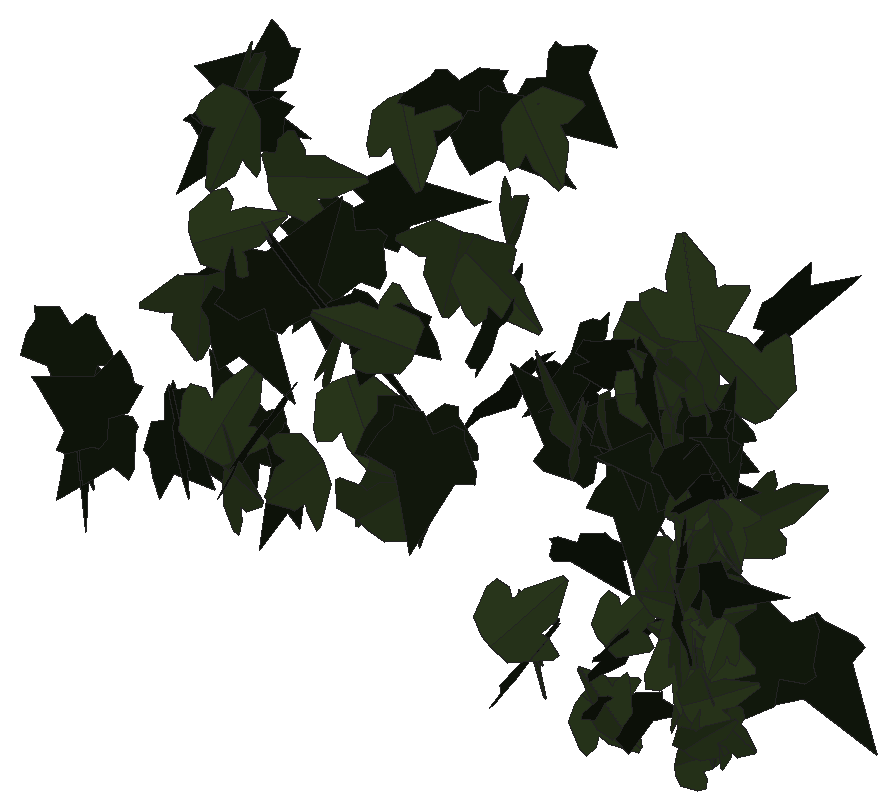
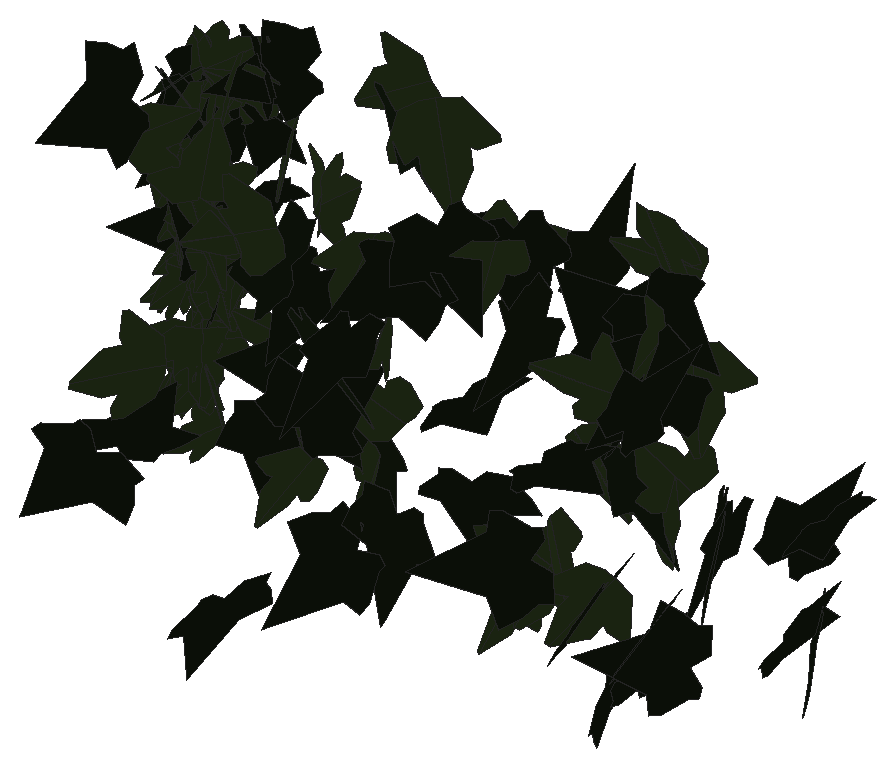
# SketchUp Ruby script. Lengths in inches.
U = 1.inch
M = Sketchup.active_model
def pt(a) = Geom::Point3d.new(a.map { |v| v * U })
def face(e, loops, mat)
  f = e.add_face(loops[0].map { |a| pt(a) })
  loops[1..].each { |l| e.add_face(l.map { |a| pt(a) }).erase! }
  f.material = f.back_material = mat if mat
  f
end
# faces: each face lists its corners as indices into pts; further lists are holes
def faces(e, pts, list, mat = nil) = list.each { |f| face(e, (f[0].is_a?(Array) ? f : [f]).map { |l| l.map { |i| pts[i] } }, mat) }
# xy, xz, yz: faces in a plane at the given z, y or x. An outline is a flat list of corners, or four numbers for a rectangle; further outlines are holes
def ring(l) = l.size == 4 ? [[l[0], l[1]], [l[2], l[1]], [l[2], l[3]], [l[0], l[3]]] : l.each_slice(2).to_a
def flat(e, list, mat, &to3) = list.each { |f| face(e, (f[0].is_a?(Array) ? f : [f]).map { |l| ring(l).map { |u, v| to3.(u, v) } }, mat) }
def xy(e, z, list, mat = nil) = flat(e, list, mat) { |x, y| [x, y, z] }
def xz(e, y, list, mat = nil) = flat(e, list, mat) { |x, z| [x, y, z] }
def yz(e, x, list, mat = nil) = flat(e, list, mat) { |y, z| [x, y, z] }
def lines(e, pts, list) = list.each { |a, b| e.add_line(pt(pts[a]), pt(pts[b])) }
# prism: a flat outline (further loops are holes) pulled along v
def prism(e, loops, v, mat = nil)
  f = face(e, loops, mat); d = Geom::Vector3d.new(v.map { |x| x * U })
  f.pushpull(f.normal.samedirection?(d) ? d.length : -d.length)
end
def box(e, o, s, mat = nil) = prism(e, [[o, [o[0] + s[0], o[1], o[2]], [o[0] + s[0], o[1] + s[1], o[2]], [o[0], o[1] + s[1], o[2]]]], [0, 0, s[2]], mat)
def at(x, y, z, deg = 0) = Geom::Transformation.translation(pt([x, y, z])) * Geom::Transformation.rotation(ORIGIN, Z_AXIS, deg.degrees)
def axes(o, x, y, z) = Geom::Transformation.new([*x, 0, *y, 0, *z, 0, *pt(o).to_a, 1])
def part(name) = M.definitions.add(name)
# library, detail: a bought-in or finely detailed component or shape, given as its bounding box
def library(name, o, s) = part(name).tap { |d| box(d.entities, o, s) }
def detail(e, o, s) = box(e.add_group.entities, o, s)
def put(e, d, t, mat = nil) = e.add_instance(d, t).tap { |i| i.material = mat if mat }
def group(e, t, mat = nil) = e.add_group.tap { |g| g.transformation = t; g.material = mat if mat }.entities
root = M.entities
M.materials.add("efeu1").color = [18, 25, 13]
M.materials.add("efeu2").color = [43, 57, 29]
c1 = part("ivyleaf_9")
p = [[1.54,2.16,1.25],[1.36,2.04,1.19],[-0.21,0.99,0.68],[-0.71,1.11,0.82],[-0.85,0.86,0.67],[-0.8,0.17,0.21],
  [-0.9,-0.01,0.1],[-0.67,-0.16,-0.02],[-0.08,-0.08,-0.05],[-0.03,-0.6,-0.4],[0.65,-0.88,-0.66],[0.83,-0.6,-0.49],
  [1.29,-0.42,-0.43],[1.8125,-0.07,-0.26],[1.21,0.44,0.15]]
faces(c1.entities,p,[[0,1,2,3,4,5,6,7,8,9,10,11,12,13,14]],"efeu1")
c2 = part("ivyleaf_10")
p = [[0,0.5,-0.03],[-0.0625,2.02,-0.43],[-0.19,2.01,-0.46],[-0.54,1.05,-0.29],[-0.52,0.625,-0.18],[-0.83,0.76,-0.28],
  [-1.16,0.64,-0.33],[-1.15,0.33,-0.24],[-0.77,-0.39,0.02],[-0.3,-0.51,0.16],[0.04,-0.48,0.23],[-0.02,2.01,-0.4375],
  [-0.06,2.01,-0.43],[0.04,-0.49,0.23],[0.67,-0.49,0.14],[1.38,0.36,-0.2],[1.375,0.51,-0.24],[0.81,0.65,-0.19],
  [0.62,0.59,-0.15],[0.6,1.09,-0.28],[0.5,1.23,-0.31]]
faces(c2.entities,p,[[0,1,2,3,4,5,6,7,8,9,10],[11,12,0,13,14,15,16,17,18,19,20]],"efeu2")
put(root,c1,axes([583.79,128.49,183.1],[-0.12016,-0.0856,-0.79424],[0.79532,0.06246,-0.12705],[0.07487,-0.80085,0.07498]))
put(root,c1,axes([567.09,128.81,175.58],[0.13274,0.09874,0.93701],[-0.726,-0.59242,0.16528],[0.60055,-0.738,-0.00731]))
put(root,c1,axes([585.98,127.68,181.96],[0.01694,-0.04648,-0.86386],[-0.20447,0.83933,-0.04917],[0.8406,0.2051,0.00545]))
put(root,c2,axes([585.875,128.125,173.35],[-0.19771,-0.43738,0.41865],[0.32575,0.29438,0.46139],[-0.51035,0.35734,0.13231]))
put(root,c1,axes([584.82,128.85,180.61],[-0.00657,-0.61648,-0.48603],[-0.00925,-0.48595,0.61651],[-0.78498,0.01088,-0.0032]))
put(root,c2,axes([585.32,128.31,176.07],[-0.07868,0.66519,-0.09517],[-0.06743,-0.10315,-0.66524],[-0.66857,-0.06787,0.07829]))
put(root,c2,axes([585.4375,128.4,180.03],[0.15282,0.5978,-0.18121],[-0.06229,-0.17104,-0.61678],[-0.62154,0.16413,0.01726]))
put(root,c2,axes([585.41,128.08,181.9375],[-0.21257,0.57692,0.24713],[-0.17654,0.19543,-0.60806],[-0.60228,-0.26091,0.09101]))
put(root,c1,axes([583.82,128.62,179.59],[-0.30966,-0.67686,-0.20143],[0.11175,0.17021,-0.74374],[0.6973,-0.32786,0.02974]))
put(root,c1,axes([583.64,128.48,181.51],[-0.47119,-0.2718,-0.5388],[0.46489,0.27237,-0.54395],[0.38478,-0.66192,-0.00259]))
put(root,c2,axes([579.09,128.24,184.09],[0.49056,0.06294,0.91802],[0.87982,0.27263,-0.48884],[-0.26952,1.00453,0.07515]))
put(root,c2,axes([583.32,128.24,173.26],[0.3648,0.04398,0.68709],[-0.68849,0.02002,0.36426],[0.00291,-0.77767,0.04824]))
put(root,c2,axes([585.92,128.26,182.72],[-0.33173,0.17249,0.58267],[-0.60038,0.00946,-0.34461],[-0.09382,-0.67041,0.14505]))
put(root,c1,axes([582.91,127.96,183.02],[0.62989,0.166,0.53267],[0.51145,0.14923,-0.65131],[-0.22295,0.81131,0.01081]))
put(root,c1,axes([584.94,128.93,176.01],[-0.07537,-0.09206,0.75222],[0.05872,-0.75436,-0.08644],[0.75555,0.04945,0.08175]))
put(root,c2,axes([585.77,128.65,179.61],[-0.17454,-0.59312,0.24394],[-0.04715,-0.24026,-0.61791],[0.63959,-0.17957,0.02102]))
put(root,c2,axes([576.07,128.78,180.8125],[0.26259,0.20311,0.97216],[-0.75178,-0.61645,0.33186],[0.64899,-0.79627,-0.00894]))
put(root,c2,axes([583.14,128.09,181.3125],[-0.51329,0.55272,0.38466],[-0.253,0.28995,-0.75422],[-0.62406,-0.57216,-0.01062]))
put(root,c2,axes([586.11,127.83,178.6],[-0.06695,-0.35913,-0.84578],[0.15964,0.83058,-0.36532],[0.90489,-0.1731,0.00188]))
put(root,c1,axes([585.9,128.125,177.66],[0.46519,0.07475,0.61592],[0.60988,0.08629,-0.4711],[-0.11395,0.76701,-0.00702]))
put(root,c2,axes([586.12,128.9,176.23],[-0.31429,-0.33866,0.44609],[0.30318,-0.53297,-0.19102],[0.47092,0.1171,0.42069]))
put(root,c2,axes([580.07,128.08,174.52],[0.5783,0.29041,-0.71908],[0.6424,0.3231,0.64713],[0.43444,-0.86435,0.0003]))
put(root,c2,axes([585,128.61,182.77],[-0.40556,-0.01263,-0.64047],[-0.63762,-0.06496,0.40504],[-0.06162,0.75528,0.02413]))
put(root,c2,axes([586.05,128.65,179.375],[-0.32491,0.26349,-0.59248],[0.48392,-0.34257,-0.41773],[-0.4316,-0.58245,-0.02234]))
put(root,c2,axes([585.87,128.97,178.53],[0.0214,-0.3494,0.59165],[0.0168,-0.59149,-0.34992],[0.68691,0.02536,-0.00988]))
put(root,c1,axes([585.87,128.88,182.17],[0.08752,-0.76967,0.07275],[0.25105,-0.04095,-0.73528],[0.7312,0.10619,0.24374]))
put(root,c2,axes([585.21,128.68,180.78],[0.09287,0.67958,-0.25538],[-0.09271,-0.24425,-0.68368],[-0.72004,0.1191,0.05509]))
put(root,c1,axes([585.93,128.42,181.58],[-0.2135,0.72701,-0.20114],[0.05702,-0.19288,-0.75771],[-0.75217,-0.22098,-0.00035]))
put(root,c1,axes([582.31,128.18,177.65],[0.70439,0.47853,-0.09165],[-0.07942,-0.04618,-0.85154],[-0.48071,0.70883,0.00639]))
put(root,c2,axes([585.92,128.2,174.51],[-0.13819,-0.20304,0.70227],[0.37275,0.59525,0.24544],[-0.62886,0.39744,-0.00884]))
put(root,c2,axes([583.69,128.44,182.26],[0.19468,-0.06436,-0.74939],[0.74945,0.08217,0.18764],[0.06371,-0.7699,0.08267]))
put(root,c1,axes([580.65,128.21,173.8125],[-0.34624,0.8815,0.13587],[-0.06915,0.11878,-0.94683],[-0.88922,-0.35247,0.02073]))
put(root,c2,axes([584.99,128.96,176.42],[-0.22187,-0.17533,-0.61383],[-0.49851,-0.35834,0.28254],[-0.39877,0.54553,-0.01169]))
put(root,c2,axes([583.39,128.18,175.6],[0.31107,0.34111,-0.62235],[0.41935,0.45985,0.46165],[0.57256,-0.52213,0]))
put(root,c2,axes([585,128.61,178.02],[-0.70386,-0.09288,0.35332],[-0.34475,-0.08487,-0.7091],[0.12086,-0.78298,0.03495]))
put(root,c2,axes([585.74,128.4,181.54],[-0.02514,0.61002,0.22863],[-0.24755,0.20269,-0.56803],[-0.60259,-0.10871,0.22382]))
put(root,c1,axes([573.06,129.07,181.18],[0.7437,-0.64796,0.21808],[-0.15515,0.15387,0.98628],[-0.66584,-0.75959,0.01376]))
put(root,c2,axes([584.78,128.27,181.59],[-0.06962,-0.31215,-0.57435],[0.12471,0.56064,-0.31982],[0.64169,-0.14283,-0.00016]))
put(root,c1,axes([585.9,128.11,180.3],[0.36826,0.52135,0.42899],[0.25734,0.34338,-0.63822],[-0.62419,0.44915,-0.01002]))
put(root,c2,axes([570.74,128.39,182.05],[0.27982,0.08284,-0.88496],[0.82809,0.31279,0.29112],[0.32293,-0.87386,0.02031]))
put(root,c2,axes([585.875,128.93,174.04],[0.07913,-0.68134,0.1746],[0.2311,-0.14077,-0.65402],[0.66431,0.13013,0.20672]))
put(root,c2,axes([585.79,128.45,175.32],[-0.47612,0.331,0.45091],[-0.3752,0.25019,-0.57983],[-0.41486,-0.60615,0.00691]))
put(root,c2,axes([585.34,128.77,175.67],[0.05747,0.06456,0.68798],[-0.67345,-0.14937,0.07028],[0.15475,-0.67402,0.05032]))
put(root,c1,axes([579.77,128.125,182.84],[-0.60602,0.28227,-0.79977],[-0.71902,0.35033,0.66847],[0.44981,0.9403,-0.00897]))
put(root,c1,axes([586.12,128.39,181.1],[-0.61001,0.45601,0.04757],[0.03476,-0.03295,0.7616],[0.45717,0.61098,0.00557]))
put(root,c2,axes([582.06,128.26,180.15],[0.24408,-0.1282,0.83626],[-0.59438,0.5934,0.26445],[-0.60206,-0.63779,0.07795]))
put(root,c1,axes([583.0625,128.18,174.75],[-0.0816,0.68765,-0.40374],[-0.04522,0.40121,0.69248],[0.79614,0.09327,-0.00205]))
put(root,c2,axes([570.63,129.15,175.02],[-0.24005,0.07296,1.05185],[1.00781,-0.30115,0.2509],[0.30986,1.03601,-0.00115]))
put(root,c2,axes([586.15,128.78,179.54],[0.53344,0.3404,0.2641],[0.22357,0.14059,-0.6328],[-0.36829,0.5784,-0.00161]))
put(root,c2,axes([583.95,128.54,177.625],[-0.11652,0.6361,0.31094],[-0.05491,0.30606,-0.64669],[-0.7059,-0.12881,-0.00103]))
put(root,c1,axes([583.33,128.61,173.42],[0.3726,0.64179,-0.29542],[-0.16179,-0.2476,-0.74196],[-0.68774,0.40595,0.0145]))
put(root,c2,axes([584.45,128.625,182.84],[-0.43751,0.59384,0.31254],[-0.18247,0.25377,-0.7376],[-0.64578,-0.47402,-0.00333]))
put(root,c2,axes([573.35,128.85,176.3125],[0.71109,-0.24592,-0.67848],[-0.6104,0.30317,-0.74963],[0.38499,0.93491,0.06462]))
put(root,c2,axes([584.42,129.04,180.39],[0.34352,0.01138,0.67998],[0.68004,0.00251,-0.34359],[-0.00737,0.76183,-0.00903]))
put(root,c2,axes([585.98,128.85,178.53],[0.14134,-0.59759,-0.2674],[-0.06972,0.25826,-0.61403],[0.65096,0.15741,-0.00771]))
put(root,c2,axes([585.3125,128.71,178.48],[0.26496,0.59256,0.30134],[0.08749,0.29049,-0.64815],[-0.65899,0.27681,0.03511]))
put(root,c1,axes([565.61,129.35,177.21],[-0.01117,-0.90154,-0.05999],[0.00491,0.05993,-0.9016],[0.90352,-0.01147,0.00415]))
put(root,c1,axes([575.63,128.86,181.43],[0.52302,0.51429,-0.71464],[-0.49877,-0.51191,-0.73343],[-0.72556,0.72263,-0.01096]))
put(root,c2,axes([586.01,128.51,177.42],[0.01196,-0.14767,-0.67473],[0.11918,0.66515,-0.14346],[0.68034,-0.11392,0.03699]))
put(root,c2,axes([584.81,129.07,174.23],[0.4648,-0.49605,-0.07245],[-0.04964,0.05277,-0.67978],[0.49885,0.46744,-0.00014]))
put(root,c2,axes([585.3125,128.58,172.47],[0.01761,0.01773,0.67581],[-0.00397,0.67603,-0.01763],[-0.67603,-0.00351,0.01771]))
put(root,c2,axes([585.08,129.08,175.21],[0.79303,0.68295,0.06639],[0.04965,0.04408,-1.04657],[-0.68437,0.79458,0.001]))
put(root,c2,axes([585.4,128.75,173.9],[-0.12072,-0.35647,-0.56093],[0.33329,0.46077,-0.36454],[0.575,-0.34191,0.09354]))
put(root,c2,axes([584.64,129.01,177.25],[0.66162,0.18067,-0.19956],[-0.24958,0.21324,-0.63438],[-0.10089,0.65733,0.26065]))
put(root,c2,axes([585.55,129.04,180.2],[0.5459,0.2007,-0.42642],[-0.46991,0.18189,-0.51596],[-0.03604,0.66839,0.26845]))
put(root,c2,axes([584.93,128.72,178.8],[0.01165,0.21733,0.71636],[-0.60985,0.41826,-0.11697],[-0.43415,-0.58169,0.18354]))
put(root,c2,axes([577.78,129.18,183.88],[-0.98814,-0.47344,0.28694],[-0.24178,-0.15906,-1.09505],[0.49802,-1.01659,0.0377]))
put(root,c2,axes([569.83,129.22,179.875],[-0.68243,-0.84989,0.07287],[-0.04369,-0.05837,-1.08996],[0.85189,-0.68382,0.00248]))
put(root,c2,axes([585.82,129,180.79],[-0.46845,0.48772,0.16867],[-0.1122,0.12609,-0.67622],[-0.50372,-0.48166,-0.00624]))
put(root,c2,axes([585.85,128.77,176.68],[-0.05846,-0.14157,-0.65994],[0.29327,0.59129,-0.15282],[0.60791,-0.29886,0.01026]))
put(root,c2,axes([581.32,128.92,180.33],[-0.42364,0.39933,-0.75901],[-0.60181,0.46475,0.58041],[0.61106,0.73456,0.0454]))
put(root,c2,axes([570.46,128.79,176.29],[0.51033,0.60104,-0.65119],[0.42213,0.49583,0.78846],[0.77916,-0.66229,-0.00066]))
put(root,c2,axes([586.22,129.04,173.52],[0.14698,-0.48984,-0.401],[0.1806,0.427,-0.45541],[0.60673,-0.00845,0.2327]))
put(root,c1,axes([569.18,128.93,176.08],[0.44441,-0.11014,-0.90603],[-0.84941,0.31882,-0.4554],[0.33396,0.95747,0.04741]))
put(root,c1,axes([571.61,129.39,176.76],[-0.51727,0.78347,-0.3447],[0.19832,-0.28209,-0.93878],[-0.83265,-0.5539,-0.00946]))
put(root,c1,axes([568.85,129,175.9375],[0.37532,-0.38393,-0.85916],[-0.6014,0.61358,-0.53691],[0.72379,0.7089,-0.0006]))
put(root,c1,axes([585.3,128.8,178.02],[-0.00211,-0.21713,1.03863],[0.30078,0.9959,0.20881],[-1.01756,0.29483,0.05956]))
put(root,c2,axes([582.08,129.01,172.71],[0.22268,0.61298,0.58588],[0.13747,0.57164,-0.65033],[-0.83673,0.25705,0.04907]))
put(root,c2,axes([585.85,129.05,176.53],[0.08778,-0.05052,0.67471],[-0.25021,0.62971,0.0797],[-0.62863,-0.2577,0.06249]))
put(root,c2,axes([584.89,129.07,177.74],[0.02424,0.31096,-0.61771],[0.02196,0.61743,0.31169],[0.69122,-0.03052,0.01176]))
put(root,c1,axes([565.29,130.13,174.18],[0.08704,-0.00215,-1.04786],[0.97838,-0.37635,0.08204],[-0.37523,-0.98181,-0.02915]))
put(root,c1,axes([570.56,129.47,179.78],[0.52293,-0.72251,-0.61524],[-0.3161,0.52973,-0.89076],[0.89477,0.60939,0.04488]))
put(root,c1,axes([565.82,130.62,174.39],[-0.18889,-0.82239,0.63797],[-0.15633,-0.61862,-0.84374],[1.02903,-0.24494,-0.01108]))
put(root,c1,axes([575.99,130.32,177.4],[-0.27265,-0.94728,0.00725],[0.01091,-0.01069,-0.98564],[0.94724,-0.27254,0.01344]))
put(root,c2,axes([579.43,129.67,173.88],[-0.6706,0.74452,-0.04122],[0.02347,-0.03433,-1.00199],[-0.74529,-0.67099,0.00554]))
put(root,c1,axes([571.65,129.38,180.07],[-0.29172,-0.26332,1.0162],[0.92685,0.43063,0.37765],[-0.49291,0.96557,0.1087]))
put(root,c1,axes([581.58,130.16,179.03],[0.67725,-0.66916,0.44254],[0.31763,-0.30817,-0.95207],[0.7367,0.74803,0.00366]))
put(root,c1,axes([574.07,129.73,179.96],[0.97546,-0.13492,-0.2079],[-0.20613,0.02714,-0.98475],[0.13761,0.997,-0.00132]))
put(root,c2,axes([569.99,130.31,184.19],[0.99711,-0.36879,-0.24772],[-0.22464,0.10659,-1.06291],[0.38329,1.02188,0.02147]))
put(root,c2,axes([585.48,131.27,181.66],[0.62008,0.26001,0.85246],[-0.78333,-0.33632,0.67238],[0.42509,-0.99904,-0.00448]))
put(root,c2,axes([573.3,131.33,173.92],[-0.58949,-0.48417,0.65374],[0.61766,0.25903,0.7488],[-0.52943,0.8413,0.14568]))
put(root,c1,axes([568.95,132.02,183.32],[-0.05624,0.43277,-0.84754],[0.03163,-0.84769,-0.43495],[-0.95111,-0.05378,0.03565]))
put(root,c1,axes([585.39,131.88,173.52],[-0.86332,-0.62694,0.10491],[0.09024,0.05427,1.06691],[-0.62922,0.86798,0.00907]))
put(root,c1,axes([574.26,132.18,176.43],[-0.61272,-0.65303,-0.50074],[0.33874,0.3688,-0.89547],[0.74996,-0.70011,-0.00464]))
put(root,c2,axes([582.64,132.23,181.05],[1.00882,-0.37496,-0.0712],[-0.06703,0.02404,-1.07625],[0.37573,1.01104,-0.00081]))
put(root,c2,axes([580.84,132.2,181.18],[0.35672,0.05065,1.00626],[0.89161,0.48126,-0.3403],[-0.46921,0.953,0.11837]))
put(root,c2,axes([582.29,132.54,182.02],[0.68814,0.79262,0.05381],[-0.03525,-0.04067,1.04966],[0.79367,-0.68904,-0.00004]))
put(root,c1,axes([569.14,133.38,173.13],[0.13333,-0.15782,-0.98314],[0.77944,-0.60072,0.20214],[-0.61963,-0.78961,0.04273]))
put(root,c1,axes([585.21,131.84,183.07],[0.27278,0.51636,0.92297],[0.47839,0.78984,-0.58326],[-0.94321,0.54994,-0.02891]))
put(root,c1,axes([568.54,132.86,173.14],[-0.41967,-0.82739,0.35569],[0.15362,0.3209,0.92771],[-0.88741,0.44684,-0.00762]))
put(root,c1,axes([578.89,132.95,176.79],[0.22937,-0.00539,1.00933],[-0.96462,0.30352,0.22083],[-0.29712,-0.98956,0.06224]))
put(root,c1,axes([578.82,132.88,179.48],[-0.80259,0.59372,-0.03443],[0.02043,-0.03028,-0.99825],[-0.59436,-0.80276,0.01218]))
put(root,c2,axes([572.55,132.42,174.41],[-0.0352,-0.59204,-0.8241],[0.17791,0.80822,-0.58823],[0.999,-0.16479,0.07572]))
put(root,c1,axes([585.26,133.08,173.78],[-0.26751,-0.26465,-1.02395],[0.72687,0.72121,-0.3763],[0.76823,-0.77453,-0.00052]))
put(root,c2,axes([569.35,133.01,181.11],[-0.19451,-0.09506,0.98352],[0.82329,0.5387,0.21489],[-0.54639,0.84555,-0.02633]))
put(root,c2,axes([571.09,133.32,175.49],[0.83755,0.30136,0.48768],[0.45856,0.16602,-0.89011],[-0.34406,0.95486,0.00085]))
put(root,c2,axes([572.67,133.4,183.88],[0.5037,0.80992,0.16445],[0.08668,0.13975,-0.95377],[-0.82189,0.51111,0.0002]))
put(root,c2,axes([568.02,132.93,182.88],[0.05623,-0.09961,0.98424],[-0.56721,0.80445,0.11382],[-0.81051,-0.56987,-0.01137]))
put(root,c2,axes([570.45,133.67,176.96],[0.36312,-0.90909,-0.12377],[-0.04947,0.11352,-0.97893],[0.91615,0.36646,-0.0038]))
put(root,c1,axes([567.25,132.99,182.26],[0.73829,0.54308,0.36462],[0.29008,0.22099,-0.9165],[-0.58629,0.79321,0.0057]))
put(root,c1,axes([570.3,134.33,179.34],[-0.55374,-0.77052,0.15859],[-0.09045,-0.13029,-0.94885],[0.78145,-0.56107,0.00255]))
put(root,c2,axes([583.79,132.97,176.65],[0.11356,-0.2095,1.0564],[0.06121,1.06179,0.20399],[-1.07523,0.03832,0.12319]))
put(root,c1,axes([573.59,134.33,184.64],[0.10672,0.71295,-0.66483],[-0.06095,-0.66262,-0.72036],[-0.97293,0.11971,-0.02779]))
put(root,c1,axes([567.05,135.25,181.89],[0.02005,-0.01733,0.94339],[-0.62966,-0.703,0.00047],[0.70272,-0.62942,-0.0265]))
put(root,c1,axes([566.66,134.79,176.26],[0.4553,-0.8092,-0.15571],[-0.07612,0.13584,-0.92849],[0.82052,0.46162,0.00026]))
put(root,c2,axes([575.39,133.99,181.33],[0.12408,-0.08133,-0.97729],[-0.20507,0.96115,-0.10602],[0.95898,0.21606,0.10378]))
put(root,c1,axes([574.68,134.61,176.4],[0.04394,0.95421,0.22388],[0.0076,0.22376,-0.95522],[-0.98009,0.04451,0.00263]))
put(root,c1,axes([573.9,134.93,183.62],[-0.06587,-0.06032,-0.97559],[0.55225,0.80448,-0.08703],[0.80649,-0.55581,-0.02009]))
put(root,c1,axes([565.53,134.89,175.625],[0.43252,0.10417,0.82238],[0.79243,0.22035,-0.44468],[-0.24335,0.90268,0.01365]))
put(root,c2,axes([575.22,135.1,183.91],[0.23113,0.90752,0.32721],[0.09692,0.31293,-0.93636],[-0.95983,0.25014,-0.01576]))
put(root,c1,axes([567.99,136.15,176.36],[0.38947,-0.67102,-0.55582],[0.30127,-0.46756,0.77557],[-0.81758,-0.49195,0.02102]))
put(root,c2,axes([567.76,135.38,177.12],[-0.74333,-0.19567,-0.54965],[0.52988,0.14619,-0.76864],[0.2442,-0.91284,-0.00528]))
put(root,c1,axes([574.8125,136.15,176.1],[0.92334,0.31164,0.17088],[0.15943,0.06198,-0.97448],[-0.31765,0.93697,0.00762]))
put(root,c1,axes([568.67,137.1,178.43],[0.26366,0.41927,-0.86319],[0.24474,0.83619,0.48091],[0.92789,-0.33969,0.11843]))
put(root,c1,axes([573.66,137.76,183.27],[0.21386,-0.40455,-0.93147],[-0.38303,0.84947,-0.45687],[0.94053,0.43793,0.02574]))
put(root,c1,axes([576.86,138.54,175.05],[0.1107,-0.93705,-0.4706],[-0.05488,0.46739,-0.94357],[1.04715,0.12356,0.0003]))
